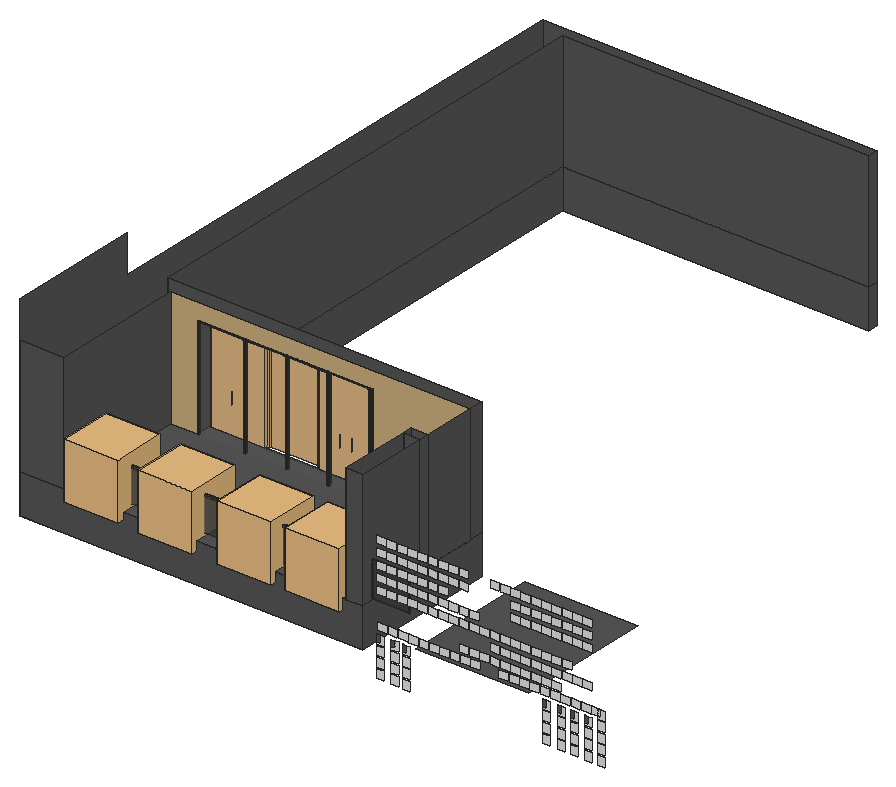
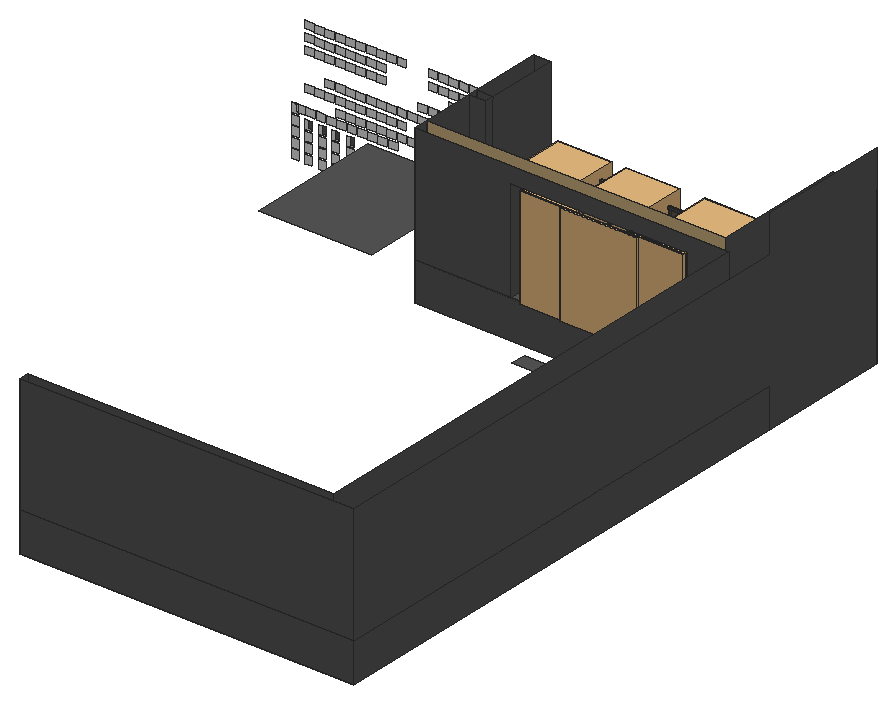
# SketchUp Ruby script. Lengths in inches.
U = 1.inch
M = Sketchup.active_model
def pt(a) = Geom::Point3d.new(a.map { |v| v * U })
def face(e, loops, mat)
  f = e.add_face(loops[0].map { |a| pt(a) })
  loops[1..].each { |l| e.add_face(l.map { |a| pt(a) }).erase! }
  f.material = f.back_material = mat if mat
  f
end
# faces: each face lists its corners as indices into pts; further lists are holes
def faces(e, pts, list, mat = nil) = list.each { |f| face(e, (f[0].is_a?(Array) ? f : [f]).map { |l| l.map { |i| pts[i] } }, mat) }
# xy, xz, yz: faces in a plane at the given z, y or x. An outline is a flat list of corners, or four numbers for a rectangle; further outlines are holes
def ring(l) = l.size == 4 ? [[l[0], l[1]], [l[2], l[1]], [l[2], l[3]], [l[0], l[3]]] : l.each_slice(2).to_a
def flat(e, list, mat, &to3) = list.each { |f| face(e, (f[0].is_a?(Array) ? f : [f]).map { |l| ring(l).map { |u, v| to3.(u, v) } }, mat) }
def xy(e, z, list, mat = nil) = flat(e, list, mat) { |x, y| [x, y, z] }
def xz(e, y, list, mat = nil) = flat(e, list, mat) { |x, z| [x, y, z] }
def yz(e, x, list, mat = nil) = flat(e, list, mat) { |y, z| [x, y, z] }
def lines(e, pts, list) = list.each { |a, b| e.add_line(pt(pts[a]), pt(pts[b])) }
# prism: a flat outline (further loops are holes) pulled along v
def prism(e, loops, v, mat = nil)
  f = face(e, loops, mat); d = Geom::Vector3d.new(v.map { |x| x * U })
  f.pushpull(f.normal.samedirection?(d) ? d.length : -d.length)
end
def box(e, o, s, mat = nil) = prism(e, [[o, [o[0] + s[0], o[1], o[2]], [o[0] + s[0], o[1] + s[1], o[2]], [o[0], o[1] + s[1], o[2]]]], [0, 0, s[2]], mat)
def at(x, y, z, deg = 0) = Geom::Transformation.translation(pt([x, y, z])) * Geom::Transformation.rotation(ORIGIN, Z_AXIS, deg.degrees)
def axes(o, x, y, z) = Geom::Transformation.new([*x, 0, *y, 0, *z, 0, *pt(o).to_a, 1])
def part(name) = M.definitions.add(name)
# library, detail: a bought-in or finely detailed component or shape, given as its bounding box
def library(name, o, s) = part(name).tap { |d| box(d.entities, o, s) }
def detail(e, o, s) = box(e.add_group.entities, o, s)
def put(e, d, t, mat = nil) = e.add_instance(d, t).tap { |i| i.material = mat if mat }
def group(e, t, mat = nil) = e.add_group.tap { |g| g.transformation = t; g.material = mat if mat }.entities
root = M.entities
M.materials.add("Glazing").color = [128, 128, 128]
M.materials["Glazing"].alpha = 0.05
M.materials.add("Powdercoating").color = [41, 44, 40]
M.materials.add("[0135_DarkGray]").color = [81, 81, 81]
M.materials.add("[Color M06]").color = [86, 86, 86]
M.materials.add("[Polished Concrete Old]").color = [229, 229, 229]
M.materials.add("[Translucent Glass Safety]").color = [204, 235, 244]
M.materials["[Translucent Glass Safety]"].alpha = 0.5
M.materials.add("[Translucent_Glass_Gray]").color = [63, 63, 63]
M.materials["[Translucent_Glass_Gray]"].alpha = 0.54
M.materials.add("[Wood Floor Light]").color = [204, 176, 127]
c1 = library("Pot+Plant",[-20.81,-17.08,-0.03],[39.86,39.43,41.33])
c2 = part("Group\#15")
xy(c2.entities,0,[[0,-55.94,0.71,45.94]])
xy(c2.entities,0.2,[[0,-55.94,0.47,45.94],[0.47,45.94,0.71,46.42]])
xy(c2.entities,2.36,[[0.47,-55.94,0.71,46.42]])
xz(c2.entities,-55.94,[[0,0,0.71,0,0.71,2.36,0.47,2.36,0.47,0.2,0,0.2]])
xz(c2.entities,45.94,[[0,0,0.71,0.2]])
xz(c2.entities,46.42,[[0.47,0.2,0.71,2.36]])
yz(c2.entities,0,[[-55.94,0,45.94,0.2]])
yz(c2.entities,0.47,[[-55.94,0.2,46.42,2.36]])
yz(c2.entities,0.71,[[-55.94,0,45.94,0,45.94,0.2,46.42,0.2,46.42,2.36,-55.94,2.36]])
c3 = part("Group\#7")
xy(c3.entities,0,[[0,-59.09,0.71,45.94]])
xy(c3.entities,0.2,[[0,-59.09,0.47,45.94],[0.47,45.94,0.71,46.42]])
xy(c3.entities,2.36,[[0.47,-59.09,0.71,46.42]])
xz(c3.entities,-59.09,[[0,0,0.71,0,0.71,2.36,0.47,2.36,0.47,0.2,0,0.2]])
xz(c3.entities,45.94,[[0,0,0.71,0.2]])
xz(c3.entities,46.42,[[0.47,0.2,0.71,2.36]])
yz(c3.entities,0,[[-59.09,0,45.94,0.2]])
yz(c3.entities,0.47,[[-59.09,0.2,46.42,2.36]])
yz(c3.entities,0.71,[[-59.09,0,45.94,0,45.94,0.2,46.42,0.2,46.42,2.36,-59.09,2.36]])
c4 = part("Group\#16")
prism(c4.entities,[[[0.47,-56.18,0.2],[0,-56.18,0.2],[0,-56.18,0],[0.71,-56.18,0],[0.71,-56.18,2.36],[0.47,-56.18,2.36]]],[0,28.68,0])
c5 = part("Group\#10")
box(c5.entities,[-0.73,0,0],[27.99,0.55,102.05])
c6 = part("Group\#18")
xy(c6.entities,0,[[0.47,-56.18,0.47,-55.47,0,-55.47,0,-28.21,1.18,-28.21,1.18,-56.18]])
xy(c6.entities,0.2,[[0.71,-56.18,1.18,-28.21],[0,-55.47,0.47,-28.21],[0.47,-28.21,0.71,-27.74]])
xy(c6.entities,2.36,[[0.47,-56.18,0.71,-27.74]])
xz(c6.entities,-56.18,[[0.47,0,1.18,0,1.18,0.2,0.71,0.2,0.71,2.36,0.47,2.36]])
xz(c6.entities,-55.47,[[0,0,0.47,0.2]])
xz(c6.entities,-28.21,[[0,0,1.18,0.2]])
xz(c6.entities,-27.74,[[0.47,0.2,0.71,2.36]])
yz(c6.entities,0,[[-55.47,0,-28.21,0.2]])
yz(c6.entities,0.47,[[-56.18,0,-55.47,0.2],[-56.18,0.2,-27.74,2.36]])
yz(c6.entities,0.71,[[-56.18,0.2,-27.74,2.36]])
yz(c6.entities,1.18,[[-56.18,0,-28.21,0.2]])
c7 = part("Group\#34")
xy(c7.entities,0,[[-20.45,0,7.76,1.22]])
xy(c7.entities,0.06,[[-20.39,0.06,7.7,1.22]])
xy(c7.entities,0.47,[[-19.98,0,7.28,0.06]])
xy(c7.entities,101.89,[[-19.98,0,7.28,0.06]])
xy(c7.entities,102.3,[[-20.39,0.06,7.7,1.22]])
xy(c7.entities,102.36,[[-20.45,0,7.76,1.22]])
xz(c7.entities,0,[[[-20.45,0,7.76,102.36],[-19.98,0.47,7.28,101.89]]])
xz(c7.entities,0.06,[[[-20.39,0.06,7.7,102.3],[-19.98,0.47,7.28,101.89]]])
xz(c7.entities,1.22,[[[-20.45,0,7.76,102.36],[-20.39,0.06,7.7,102.3]]])
yz(c7.entities,-20.45,[[0,0,1.22,102.36]])
yz(c7.entities,-20.39,[[0.06,0.06,1.22,102.3]])
yz(c7.entities,-19.98,[[0,0.47,0.06,101.89]])
yz(c7.entities,7.28,[[0,0.47,0.06,101.89]])
yz(c7.entities,7.7,[[0.06,0.06,1.22,102.3]])
yz(c7.entities,7.76,[[0,0,1.22,102.36]])
c8 = part("Group\#6")
put(c8.entities,c2,axes([27.97,0,7.875],[1,0,0],[0,0,-1],[0,1,0]),"Powdercoating")
put(c8.entities,c3,axes([0.71,0,6.8],[-1,0,0],[0,0,-0.97687],[0,1,0]),"Powdercoating")
put(c8.entities,c4,axes([-27.5,0,-38.07],[0,0,-1],[-1,0,0],[0,1,0]),"Powdercoating")
put(c8.entities,c5,at(1.12,0.35,-38.39),"Glazing")
put(c8.entities,c6,axes([-27.5,0,63.35],[0,0,1],[-1,0,0],[0,1,0]),"Powdercoating")
put(c8.entities,c7,at(20.6875,1.0625,-38.54),"Powdercoating")
c9 = part("Sliding door panels")
put(c9.entities,c8,at(-1.18,4.5,38.86))
g1 = group(c9.entities,at(84.74,4.5,38.86))
put(g1,c2,axes([-27.97,0,7.875],[-1,0,0],[0,0,-1],[0,1,0]),"Powdercoating")
put(g1,c3,axes([-0.71,0,6.8],[1,0,0],[0,0,-0.97687],[0,1,0]),"Powdercoating")
put(g1,c4,axes([27.5,0,-38.07],[0,0,-1],[1,0,0],[0,1,0]),"Powdercoating")
put(g1,c5,axes([-1.12,0.35,-38.39],[-1,0,0],[0,1,0],[0,0,1]),"Glazing")
put(g1,c6,axes([27.5,0,63.35],[0,0,1],[1,0,0],[0,1,0]),"Powdercoating")
put(g1,c7,axes([-20.6875,1.0625,-38.54],[-1,0,0],[0,1,0],[0,0,1]),"Powdercoating")
g2 = group(c9.entities,at(56.0625,4.5,38.86))
put(g2,c2,axes([-27.97,0,7.875],[-1,0,0],[0,0,-1],[0,1,0]),"Powdercoating")
put(g2,c4,axes([27.5,0,-38.07],[0,0,-1],[1,0,0],[0,1,0]),"Powdercoating")
put(g2,c5,axes([-1.12,0.35,-38.39],[-1,0,0],[0,1,0],[0,0,1]),"Glazing")
put(g2,c6,axes([27.5,0,63.35],[0,0,1],[1,0,0],[0,1,0]),"Powdercoating")
put(g2,c7,axes([-20.6875,1.0625,-38.54],[-1,0,0],[0,1,0],[0,0,1]),"Powdercoating")
g3 = group(g2,at(-0.71,0,6.8),"Powdercoating")
xy(g3,-45.34,[[0.47,0.2,0.71,2.36]])
xy(g3,-44.88,[[0,0,0.71,0.2]])
xy(g3,57.73,[[0,0,0.71,0,0.71,2.36,0.47,2.36,0.47,0.2,0,0.2]])
xz(g3,0,[[0,-44.88,0.71,57.73]])
xz(g3,0.2,[[0.47,-45.34,0.71,-44.88],[0,-44.88,0.47,57.73]])
xz(g3,2.36,[[0.47,-45.34,0.71,57.73]])
yz(g3,0,[[0,-44.88,0.2,57.73]])
yz(g3,0.47,[[0.2,-45.34,2.36,57.73]])
yz(g3,0.71,[[0.2,-45.34,2.36,-45.34,2.36,57.73,0,57.73,0,-44.88,0.2,-44.88]])
put(c9.entities,c8,axes([-33.94,4.5,38.86],[1.14218,0,0],[0,1,0],[0,0,1]))
c10 = part("sliding door")
put(c10.entities,c9,at(0,-4.5,-0.08))
c11 = library("Group14",[-64.97,9.24,0.31],[138.52,9.93,292.57])
c12 = library("Group16",[86.37,-10.76,76.46],[21.79,14.87,35.97])
c13 = library("Group22",[48.82,-10.91,0.23],[97.72,18.57,293.12])
c14 = library("Group24",[44.03,2.01,0.26],[103.73,11,292.35])
c15 = library("Group27",[-106.21,-10.76,76.46],[21.8,14.87,35.97])
c16 = library("Group35",[-145.81,2.01,0.26],[103.73,11,292.35])
c17 = library("Group33",[-144.59,-10.91,0.23],[97.72,18.57,293.12])
c18 = part("rem")
g4 = group(c18.entities,at(-145.81,-10.91,0.23))
put(g4,c11,at(145.81,10.91,-0.23))
put(g4,c12,at(145.81,10.91,-0.23))
put(g4,c13,at(145.81,10.91,-0.23))
put(g4,c14,at(145.81,10.91,-0.23))
put(g4,c15,at(145.81,10.91,-0.23))
put(g4,c16,at(145.81,10.91,-0.23))
put(g4,c17,at(145.81,10.91,-0.23))
c19 = part("Group\#81")
box(c19.entities,[0,0,0],[0.79,39.37,35.43],"[Translucent_Glass_Gray]")
c20 = part("Group\#82")
box(c20.entities,[0,0,0],[0.59,1.57,34.25])
c21 = part("Group\#85")
g5 = group(c21.entities,at(0.55,0.5,0))
put(g5,c19,axes([293.06,0,0],[0,0.84,0],[-0.92977,0,0],[0,0,1]),"[Translucent Glass Safety]")
g6 = group(g5,at(0,33.57,0),"[Translucent Glass Safety]")
box(g6,[0,0,0],[0.73,33.07,35.43],"[Translucent_Glass_Gray]")
put(g5,c19,axes([218.38,0,0],[0,0.84,0],[-0.92977,0,0],[0,0,1]),"[Translucent Glass Safety]")
put(g5,c19,axes([367.73,0,0],[0,0.84,0],[-0.92977,0,0],[0,0,1]),"[Translucent Glass Safety]")
g7 = group(g5,at(31.69,0,0),"[Translucent Glass Safety]")
box(g7,[-30.96,0,0],[30.96,0.66,35.43],"[Translucent_Glass_Gray]")
put(g5,c19,axes([255.72,0,0],[0,0.84,0],[-0.92977,0,0],[0,0,1]),"[Translucent Glass Safety]")
g8 = group(g5,at(181.04,0,0),"[Translucent Glass Safety]")
box(g8,[-36.61,0,0],[36.61,0.66,35.43],"[Translucent_Glass_Gray]")
g9 = group(g5,at(0,0.66,0),"[Translucent Glass Safety]")
box(g9,[0,0,0],[0.73,32.24,35.43],"[Translucent_Glass_Gray]")
g10 = group(g5,at(143.71,0,0),"[Translucent Glass Safety]")
box(g10,[-36.61,0,0],[36.61,0.66,35.43],"[Translucent_Glass_Gray]")
g11 = group(g5,at(69.03,0,0),"[Translucent Glass Safety]")
box(g11,[-36.61,0,0],[36.61,0.66,35.43],"[Translucent_Glass_Gray]")
g12 = group(g5,at(0,67.3,0),"[Translucent Glass Safety]")
box(g12,[0,0,0],[0.73,33.07,35.43],"[Translucent_Glass_Gray]")
put(g5,c20,axes([107.44,0.66,0],[0,1,0],[-0.92977,0,0],[0,0,1]),"[0135_DarkGray]")
put(g5,c20,axes([144.78,0.66,0],[0,1,0],[-0.92977,0,0],[0,0,1]),"[0135_DarkGray]")
put(g5,c20,axes([182.11,0.66,0],[0,1,0],[-0.92977,0,0],[0,0,1]),"[0135_DarkGray]")
put(g5,c20,axes([256.79,0.66,0],[0,1,0],[-0.92977,0,0],[0,0,1]),"[0135_DarkGray]")
put(g5,c20,axes([368.14,0.66,0],[0,1,0],[-0.92977,0,0],[0,0,1]),"[0135_DarkGray]")
put(g5,c20,axes([0.73,98.83,0],[0.92977,0,0],[0,1,0],[0,0,1]),"[0135_DarkGray]")
put(g5,c20,axes([331.46,0.66,0],[0,1,0],[-0.92977,0,0],[0,0,1]),"[0135_DarkGray]")
g13 = group(g5,at(106.37,0,0),"[Translucent Glass Safety]")
box(g13,[-36.61,0,0],[36.61,0.66,35.43],"[Translucent_Glass_Gray]")
put(g5,c19,axes([330.39,0,0],[0,0.84,0],[-0.92977,0,0],[0,0,1]),"[Translucent Glass Safety]")
put(g5,c20,axes([294.125,0.66,0],[0,1,0],[-0.92977,0,0],[0,0,1]),"[0135_DarkGray]")
put(g5,c20,axes([0.73,66.04,0],[0.92977,0,0],[0,1,0],[0,0,1]),"[0135_DarkGray]")
put(g5,c20,axes([0.73,32.31,0],[0.92977,0,0],[0,1,0],[0,0,1]),"[0135_DarkGray]")
put(g5,c20,axes([32.76,0.66,0],[0,1,0],[-0.92977,0,0],[0,0,1]),"[0135_DarkGray]")
put(g5,c20,axes([70.1,0.66,0],[0,1,0],[-0.92977,0,0],[0,0,1]),"[0135_DarkGray]")
put(g5,c20,axes([219.45,0.66,0],[0,1,0],[-0.92977,0,0],[0,0,1]),"[0135_DarkGray]")
g14 = group(c21.entities,at(0,0,34.25))
xy(g14,0,[[0,0,0,100.87,0.55,100.87,0.55,0.5,362.73,0.5,362.73,0],[362.73,0,369.35,0.5],[368.19,0.5,368.6875,1.16],[1.28,1.16,1.28,100.87,1.83,100.87,1.83,1.65,362.73,1.65,362.73,1.16],[362.73,1.16,368.19,1.65]],"[0135_DarkGray]")
xy(g14,1.18,[[368.19,0,368.6875,0.5],[368.6875,0,369.35,0.5],[0.55,0.5,0.55,100.87,1.28,100.87,1.28,1.16,362.73,1.16,362.73,0.5],[368.6875,0.5,369.35,1.16]],"[0135_DarkGray]")
xy(g14,1.97,[[0,0,362.73,0,362.73,1.65,1.83,1.65,1.83,100.87,0,100.87],[362.73,0,368.19,1.65]],"[0135_DarkGray]")
xz(g14,0,[[0,0,362.73,1.97],[362.73,0,369.35,0,369.35,1.18,368.19,1.18,368.19,1.97,362.73,1.97]],"[0135_DarkGray]")
xz(g14,0.5,[[0.55,0,1.28,1.18],[1.28,0,362.73,1.18],[362.73,0,368.19,1.18],[368.19,0,368.6875,1.18],[368.6875,0,369.35,1.18]],"[0135_DarkGray]")
xz(g14,1.16,[[1.28,0,362.73,1.18],[362.73,0,368.19,1.18]],"[0135_DarkGray]")
xz(g14,1.65,[[1.83,0,362.73,1.97],[362.73,0,368.19,1.97]],"[0135_DarkGray]")
xz(g14,100.87,[[0,0,0,1.97,1.83,1.97,1.83,0,1.28,0,1.28,1.18,0.55,1.18,0.55,0]],"[0135_DarkGray]")
yz(g14,0,[[0,0,100.87,1.97]],"[0135_DarkGray]")
yz(g14,0.55,[[0.5,0,100.87,1.18]],"[0135_DarkGray]")
yz(g14,1.28,[[1.16,0,100.87,1.18]],"[0135_DarkGray]")
yz(g14,1.83,[[1.65,0,100.87,1.97]],"[0135_DarkGray]")
yz(g14,362.73,[[0,0,0,1.97,1.65,1.97,1.65,0,1.16,0,1.16,1.18,0.5,1.18,0.5,0]],"[0135_DarkGray]")
yz(g14,368.19,[[1.16,0,1.65,0,1.65,1.97,0,1.97,0,1.18,1.16,1.18],[0.5,0,1.16,1.18]],"[0135_DarkGray]")
yz(g14,368.6875,[[0.5,0,1.16,1.18]],"[0135_DarkGray]")
yz(g14,369.35,[[0,0,0.5,1.18]],"[0135_DarkGray]")
xy(root,357.83,[[74.05,145.99,250.86,161.89]],"[Color M06]")
xy(root,377.83,[[1.28,10.05,29.53,145.99],[29.53,10.05,349.9,145.99],[1.28,145.99,1.28,675.01,340.92,675.01,340.92,665.33,29.53,665.33,29.53,161.89,349.9,161.89,349.9,145.99]],"[Color M06]")
xy(root,397.33,[[404.15,10.05,518.59,148.99]],"[Color M06]")
xy(root,417.58,[[29.53,10.05,45.84,145.99],[45.84,10.05,333.03,10.05,333.03,92.58,349.9,92.58,349.9,145.99,251.64,145.99,251.64,161.89,72.77,161.89,72.77,145.99,45.84,145.99],[333.03,10.05,349.9,82.9],[333.03,82.9,349.9,92.58],[1.28,145.99,1.28,675.01,340.92,675.01,340.92,665.33,29.53,665.33,29.53,161.89,72.77,161.89,72.77,145.99],
  [251.64,145.99,349.9,161.89]],"[Color M06]")
xz(root,10.05,[[1.28,377.83,349.9,417.58],[364.31,390.38,367.52,397.24],[378.93,390.38,382.14,397.24],[390.99,390.38,394.21,397.24],[532.99,390.38,536.21,397.24],
  [548.43,390.38,551.64,397.24],[561.81,390.38,565.02,397.24],[575.62,390.38,578.83,397.24],[1.28,417.58,45.84,537.58],[333.03,417.58,349.9,537.58]],"[Color M06]")
xz(root,10.05,[[364.31,356.74,371.62,365.74],[378.93,356.74,386.24,365.74],[390.99,356.74,398.31,365.74],[532.99,356.74,540.31,365.74],[548.43,356.74,555.74,365.74],
  [561.81,356.74,569.12,365.74],[575.62,356.74,582.93,365.74],[589.18,356.91,596.49,365.91],[364.31,367.24,371.62,376.24],[378.93,367.24,386.24,376.24],
  [390.99,367.24,398.31,376.24],[532.99,367.24,540.31,376.24],[548.43,367.24,555.74,376.24],[561.81,367.24,569.12,376.24],[575.62,367.24,582.93,376.24],
  [589.18,367.41,596.49,376.41],[364.31,377.74,371.62,386.74],[378.93,377.74,386.24,386.74],[390.99,377.74,398.31,386.74],[532.99,377.74,540.31,386.74],
  [548.43,377.74,555.74,386.74],[561.81,377.74,569.12,386.74],[575.62,377.74,582.93,386.74],[589.18,377.91,596.49,386.91],[364.31,388.24,371.62,388.24,371.62,397.24,367.52,397.24,367.52,390.38,364.31,390.38],
  [378.93,388.24,386.24,388.24,386.24,397.24,382.14,397.24,382.14,390.38,378.93,390.38],[390.99,388.24,398.31,388.24,398.31,397.24,394.21,397.24,394.21,390.38,390.99,390.38],[532.99,388.24,540.31,388.24,540.31,397.24,536.21,397.24,536.21,390.38,532.99,390.38],[548.43,388.24,555.74,388.24,555.74,397.24,551.64,397.24,551.64,390.38,548.43,390.38],[561.81,388.24,569.12,388.24,569.12,397.24,565.02,397.24,565.02,390.38,561.81,390.38],
  [575.62,388.24,582.93,388.24,582.93,397.24,578.83,397.24,578.83,390.38,575.62,390.38],[589.18,388.41,596.49,397.41],[589.18,398.91,596.49,398.91,596.49,407.91,592.39,407.91,592.39,401.04,589.18,401.04],[365.64,401.04,374.64,408.36],[376.14,401.04,385.14,408.36],
  [386.64,401.04,395.64,408.36],[397.14,401.04,406.14,408.36],[407.64,401.04,416.64,408.36],[418.14,401.04,427.14,408.36],[428.64,401.04,437.64,408.36],
  [439.14,401.04,448.14,408.36],[449.64,401.04,458.64,408.36],[460.14,401.04,469.14,408.36],[488.89,401.04,497.89,408.36],[499.39,401.04,508.39,408.36],
  [509.89,401.04,518.89,408.36],[520.39,401.04,529.39,408.36],[530.89,401.04,539.89,408.36],[541.39,401.04,550.39,408.36],[551.89,401.04,560.89,408.36],
  [562.39,401.04,571.39,408.36],[572.89,401.04,581.89,408.36],[583.39,401.04,589.18,401.04,589.18,407.91,592.39,407.91,592.39,408.36,583.39,408.36],[589.18,401.04,592.39,407.91],[448.36,410.43,457.36,417.74],
  [458.86,410.43,467.86,417.74],[469.36,410.43,478.36,417.74],[479.86,410.43,488.86,417.74],[490.36,410.43,499.36,417.74],[500.86,410.43,509.86,417.74],
  [511.36,410.43,520.36,417.74],[521.86,410.43,530.86,417.74],[532.36,410.43,541.36,417.74],[542.86,410.43,551.86,417.74],[479.86,422.31,488.86,429.62],
  [490.36,422.31,499.36,429.62],[500.86,422.31,509.86,429.62],[511.36,422.31,520.36,429.62],[521.86,422.31,530.86,429.62],[532.36,422.31,541.36,429.62],
  [542.86,422.31,551.86,429.62],[553.36,422.31,562.36,429.62],[563.86,422.31,572.86,429.62],[574.36,422.31,583.36,429.62],[364.36,433.87,373.36,441.18],
  [374.86,433.87,383.86,441.18],[385.36,433.87,394.36,441.18],[395.86,433.87,404.86,441.18],[406.36,433.87,415.36,441.18],[416.86,433.87,425.86,441.18],
  [427.36,433.87,436.36,441.18],[437.86,433.87,446.86,441.18],[448.36,433.87,457.36,441.18],[458.86,433.87,467.86,441.18],[469.36,433.87,478.36,441.18],
  [479.86,433.87,488.86,441.18],[490.36,433.87,499.36,441.18],[500.86,433.87,509.86,441.18],[511.36,433.87,520.36,441.18],[521.86,433.87,530.86,441.18],
  [532.36,433.87,541.36,441.18],[542.86,433.87,551.86,441.18],[553.36,433.87,562.36,441.18],[364.36,445.43,373.36,452.75],[374.86,445.43,383.86,452.75],
  [385.36,445.43,394.36,452.75],[395.86,445.43,404.86,452.75],[406.36,445.43,415.36,452.75],[416.86,445.43,425.86,452.75],[427.36,445.43,436.36,452.75],
  [437.86,445.43,446.86,452.75],[448.36,445.43,457.36,452.75],[458.86,445.43,467.86,452.75],[364.36,457,373.36,464.31],[374.86,457,383.86,464.31],
  [385.36,457,394.36,464.31],[395.86,457,404.86,464.31],[406.36,457,415.36,464.31],[416.86,457,425.86,464.31],[427.36,457,436.36,464.31],
  [500.86,457,509.86,464.31],[511.36,457,520.36,464.31],[521.86,457,530.86,464.31],[532.36,457,541.36,464.31],[542.86,457,551.86,464.31],
  [553.36,457,562.36,464.31],[563.86,457,572.86,464.31],[574.36,457,583.36,464.31],[364.36,468.43,373.36,475.75],[374.86,468.43,383.86,475.75],
  [385.36,468.43,394.36,475.75],[395.86,468.43,404.86,475.75],[406.36,468.43,415.36,475.75],[416.86,468.43,425.86,475.75],[427.36,468.43,436.36,475.75],
  [437.86,468.43,446.86,475.75],[448.36,468.43,457.36,475.75],[500.86,468.43,509.86,475.75],[511.36,468.43,520.36,475.75],[521.86,468.43,530.86,475.75],
  [532.36,468.43,541.36,475.75],[542.86,468.43,551.86,475.75],[553.36,468.43,562.36,475.75],[563.86,468.43,572.86,475.75],[574.36,468.43,583.36,475.75],
  [364.36,479.87,373.36,487.18],[374.86,479.87,383.86,487.18],[385.36,479.87,394.36,487.18],[395.86,479.87,404.86,487.18],[406.36,479.87,415.36,487.18],
  [416.86,479.87,425.86,487.18],[427.36,479.87,436.36,487.18],[437.86,479.87,446.86,487.18],[448.36,479.87,457.36,487.18],[500.86,479.87,509.86,487.18],
  [511.36,479.87,520.36,487.18],[521.86,479.87,530.86,487.18],[532.36,479.87,541.36,487.18],[542.86,479.87,551.86,487.18],[553.36,479.87,562.36,487.18],
  [563.86,479.87,572.86,487.18],[574.36,479.87,583.36,487.18],[479.86,480,488.86,487.31],[490.36,480,499.36,487.31]],"[Polished Concrete Old]")
xz(root,82.9,[[333.03,417.58,349.9,537.58]],"[Color M06]")
xz(root,92.58,[[333.03,417.58,349.9,537.58]],"[Color M06]")
xz(root,145.99,[[1.28,377.83,29.53,417.58]],"[Color M06]")
xz(root,145.99,[[45.84,417.58,72.77,417.58,72.77,521.33,251.64,521.33,251.64,417.58,349.9,417.58,349.9,537.58,45.84,537.58]],"[Wood Floor Light]")
xz(root,161.89,[[29.53,377.83,349.9,417.58],[29.53,417.58,29.53,537.58,349.9,537.58,349.9,417.58,251.64,417.58,251.64,521.33,72.77,521.33,72.77,417.58]],"[Color M06]")
xz(root,665.33,[[29.53,377.83,340.92,417.58],[29.53,417.58,340.92,537.58]],"[Color M06]")
xz(root,675.01,[[1.28,377.83,340.92,417.58],[1.28,417.58,340.92,537.58]],"[Color M06]")
yz(root,1.28,[[10.05,377.83,10.05,575.71,145.99,575.71,145.99,537.58,675.01,537.58,675.01,417.58,145.99,417.58,145.99,377.83],[145.99,377.83,675.01,417.58]],"[Color M06]")
yz(root,29.53,[[161.89,377.83,665.33,417.58],[161.89,417.58,665.33,537.58]],"[Color M06]")
yz(root,45.84,[[10.05,417.58,145.99,537.58]],"[Color M06]")
yz(root,72.77,[[145.99,417.58,161.89,521.33]],"[Color M06]")
yz(root,251.64,[[145.99,417.58,161.89,521.33]],"[Color M06]")
yz(root,333.03,[[10.05,417.58,82.9,537.58],[82.9,417.58,92.58,537.58]],"[Color M06]")
yz(root,340.92,[[665.33,377.83,675.01,417.58],[665.33,417.58,675.01,537.58]],"[Color M06]")
yz(root,349.9,[[10.05,377.83,161.89,417.58],[10.05,417.58,82.9,537.58],[82.9,417.58,92.58,537.58],[92.58,417.58,145.99,537.58],[145.99,417.58,161.89,537.58]],"[Color M06]")
put(root,c1,axes([153.75,28.99,407.47],[1.38,0,0],[0,1.38,0],[0,0,1.38]))
put(root,c1,axes([233.63,28.99,407.47],[1.38,0,0],[0,1.38,0],[0,0,1.38]))
put(root,c1,axes([302.82,28.99,407.47],[1.38,0,0],[0,1.38,0],[0,0,1.38]))
put(root,c1,axes([79.25,26.8,410.5],[1.38,0,0],[0,1.38,0],[0,0,1.38]))
put(root,c10,axes([122.98,145.99,412.81],[1.47956,0,0],[0,1,0],[0,0,1.05053]),"[Color M06]")
put(root,c18,axes([155.59,163.96,417.55],[0.568,0,0],[0,0.19,0],[0,0,0.35379]),"[Color M06]")
put(root,c21,axes([20.7,20.11,419.63],[0.99859,0,0],[0,1,0],[0,0,1]),"[Color M06]")
